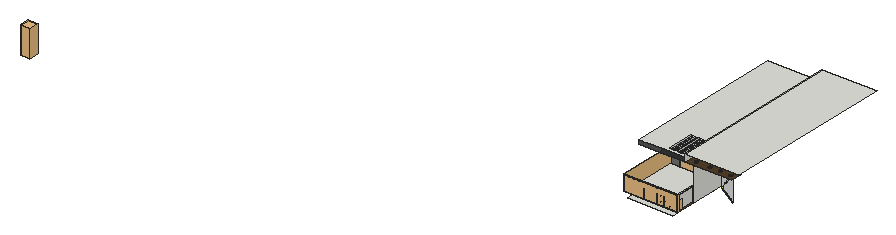
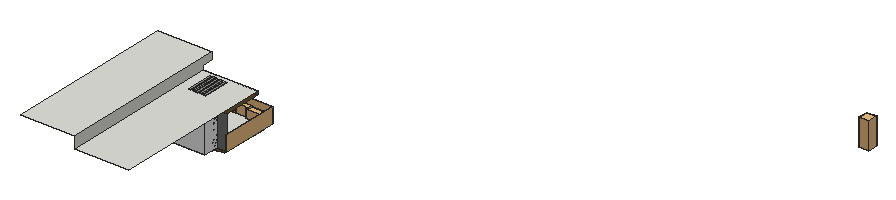
# SketchUp Ruby script. Lengths in inches.
U = 1.inch
M = Sketchup.active_model
def pt(a) = Geom::Point3d.new(a.map { |v| v * U })
def face(e, loops, mat)
  f = e.add_face(loops[0].map { |a| pt(a) })
  loops[1..].each { |l| e.add_face(l.map { |a| pt(a) }).erase! }
  f.material = f.back_material = mat if mat
  f
end
# faces: each face lists its corners as indices into pts; further lists are holes
def faces(e, pts, list, mat = nil) = list.each { |f| face(e, (f[0].is_a?(Array) ? f : [f]).map { |l| l.map { |i| pts[i] } }, mat) }
# xy, xz, yz: faces in a plane at the given z, y or x. An outline is a flat list of corners, or four numbers for a rectangle; further outlines are holes
def ring(l) = l.size == 4 ? [[l[0], l[1]], [l[2], l[1]], [l[2], l[3]], [l[0], l[3]]] : l.each_slice(2).to_a
def flat(e, list, mat, &to3) = list.each { |f| face(e, (f[0].is_a?(Array) ? f : [f]).map { |l| ring(l).map { |u, v| to3.(u, v) } }, mat) }
def xy(e, z, list, mat = nil) = flat(e, list, mat) { |x, y| [x, y, z] }
def xz(e, y, list, mat = nil) = flat(e, list, mat) { |x, z| [x, y, z] }
def yz(e, x, list, mat = nil) = flat(e, list, mat) { |y, z| [x, y, z] }
def lines(e, pts, list) = list.each { |a, b| e.add_line(pt(pts[a]), pt(pts[b])) }
# prism: a flat outline (further loops are holes) pulled along v
def prism(e, loops, v, mat = nil)
  f = face(e, loops, mat); d = Geom::Vector3d.new(v.map { |x| x * U })
  f.pushpull(f.normal.samedirection?(d) ? d.length : -d.length)
end
def box(e, o, s, mat = nil) = prism(e, [[o, [o[0] + s[0], o[1], o[2]], [o[0] + s[0], o[1] + s[1], o[2]], [o[0], o[1] + s[1], o[2]]]], [0, 0, s[2]], mat)
def at(x, y, z, deg = 0) = Geom::Transformation.translation(pt([x, y, z])) * Geom::Transformation.rotation(ORIGIN, Z_AXIS, deg.degrees)
def axes(o, x, y, z) = Geom::Transformation.new([*x, 0, *y, 0, *z, 0, *pt(o).to_a, 1])
def part(name) = M.definitions.add(name)
# library, detail: a bought-in or finely detailed component or shape, given as its bounding box
def library(name, o, s) = part(name).tap { |d| box(d.entities, o, s) }
def detail(e, o, s) = box(e.add_group.entities, o, s)
def put(e, d, t, mat = nil) = e.add_instance(d, t).tap { |i| i.material = mat if mat }
def group(e, t, mat = nil) = e.add_group.tap { |g| g.transformation = t; g.material = mat if mat }.entities
root = M.entities
M.materials.add("Concrete White 02 100cm").color = [237, 237, 237]
M.materials.add("Marble White SSS 100cm").color = [222, 222, 222]
M.materials.add("Wood Planks Pecan 33-81 150cm").color = [83, 63, 40]
M.materials.add("[Color E05]").color = [239, 239, 0]
M.materials["[Color E05]"].alpha = 0.89
M.materials.add("[Color E05]1").color = [255, 255, 0]
M.materials.add("[Color M05]").color = [114, 114, 114]
M.materials.add("[Color M06]").color = [86, 86, 86]
M.materials.add("[Color M07]").color = [58, 58, 58]
c1 = library("Planted window box",[0,0,0],[56.02,15.3,25.28])
c2 = library("Group\#2",[0,0,0],[118.08,13.29,95.4])
c3 = library("My+Glass_Railing",[-0.1,0,0],[149.63,2.52,40.9])
c4 = library("My+Glass_Railing\#1",[-0.1,0,0],[157.36,2.52,40.9])
c5 = library("30",[-486.49,477.14,411.4],[26.62,27.13,73.11])
xy(root,259.1,[[12.28,0,137.25,16.25]])
xy(root,259.1,[[[12.28,18.25,12.28,151.1875,30.69,151.1875,30.69,155.4375,118.84,155.4375,118.84,151.1875,137.25,151.1875,137.25,18.25],[123.17,35.85,124.16,35.9,125.11,36.2,125.95,36.74,126.62,37.48,127.08,38.36,127.29,39.33,127.24,40.33,126.9375,41.28,126.4,42.11,125.66,42.78,124.78,43.24,123.81,43.45,122.8125,43.4,121.87,43.1,121.03,42.5625,120.36,41.83,119.9,40.94,119.69,39.97,119.74,38.98,120.04,38.03,120.58,37.19,121.3125,36.52,122.2,36.07],[28.42,35.85,29.41,35.9,30.36,36.2,31.2,36.74,31.87,37.48,32.33,38.36,32.54,39.33,32.49,40.33,32.1875,41.28,31.65,42.11,30.91,42.78,30.03,43.24,29.06,43.45,28.0625,43.4,27.12,43.1,26.28,42.5625,25.61,41.83,25.15,40.94,24.94,39.97,24.99,38.98,25.29,38.03,25.83,37.19,26.5625,36.52,27.45,36.07],[60.17,35.85,61.16,35.9,62.11,36.2,62.95,36.74,63.62,37.48,64.08,38.36,64.29,39.33,64.24,40.33,63.9375,41.28,63.4,42.11,62.66,42.78,61.78,43.24,60.81,43.45,59.8125,43.4,58.87,43.1,58.03,42.5625,57.36,41.83,56.9,40.94,56.69,39.97,56.74,38.98,57.04,38.03,57.58,37.19,58.3125,36.52,59.2,36.07],[93.92,35.85,94.91,35.9,95.86,36.2,96.7,36.74,97.37,37.48,97.83,38.36,98.04,39.33,97.99,40.33,97.6875,41.28,97.15,42.11,96.41,42.78,95.53,43.24,94.56,43.45,93.5625,43.4,92.62,43.1,91.78,42.5625,91.11,41.83,90.65,40.94,90.44,39.97,90.49,38.98,90.79,38.03,91.33,37.19,92.0625,36.52,92.95,36.07]]],"Wood Planks Pecan 33-81 150cm")
xy(root,259.1,[[12.28,16.25,137.25,18.25]],"[Color E05]")
xy(root,271.39,[[0,0,149.53,0,149.53,1.46,146.53,1.46,146.53,54.0625,149.53,54.0625,149.53,200.375,27.125,200.375,27.125,159.875,0,159.875]])
xy(root,312.29,[[146.53,1.46,149.53,54.0625]])
xy(root,362.4,[[16.74,68.72,15.77,68.93,14.88,69.39,14.15,70.06,13.61,70.89,13.31,71.84,13.26,72.84,13.47,73.81,13.93,74.69,14.6,75.43,15.4375,75.97,16.38,76.27,17.38,76.32,18.35,76.1,19.24,75.65,19.97,74.98,20.51,74.14,20.8125,73.19,20.86,72.2,20.65,71.23,20.19,70.34,19.52,69.61,18.68,69.07,17.74,68.77],[37.18,68.72,36.21,68.93,35.32,69.39,34.59,70.06,34.05,70.89,33.75,71.84,33.7,72.84,33.91,73.81,34.37,74.69,35.04,75.43,35.875,75.97,36.82,76.27,37.82,76.32,38.79,76.1,39.67,75.65,40.41,74.98,40.95,74.14,41.25,73.19,41.3,72.2,41.08,71.23,40.63,70.34,39.96,69.61,39.12,69.07,38.17,68.77],[16.74,88.59,15.77,88.81,14.88,89.26,14.15,89.93,13.61,90.77,13.31,91.72,13.26,92.71,13.47,93.68,13.93,94.57,14.6,95.3,15.4375,95.84,16.38,96.14,17.38,96.19,18.35,95.98,19.24,95.52,19.97,94.85,20.51,94.02,20.8125,93.07,20.86,92.07,20.65,91.1,20.19,90.22,19.52,89.48,18.68,88.94,17.74,88.64],[37.18,88.59,36.21,88.81,35.32,89.26,34.59,89.93,34.05,90.77,33.75,91.72,33.7,92.71,33.91,93.68,34.37,94.57,35.04,95.3,35.875,95.84,36.82,96.14,37.82,96.19,38.79,95.98,39.67,95.52,40.41,94.85,40.95,94.02,41.25,93.07,41.3,92.07,41.08,91.1,40.63,90.22,39.96,89.48,39.12,88.94,38.17,88.64],[16.74,107.47,15.77,107.68,14.88,108.14,14.15,108.81,13.61,109.64,13.31,110.59,13.26,111.59,13.47,112.56,13.93,113.44,14.6,114.18,15.4375,114.72,16.38,115.02,17.38,115.07,18.35,114.85,19.24,114.4,19.97,113.73,20.51,112.89,20.8125,111.94,20.86,110.95,20.65,109.98,20.19,109.09,19.52,108.36,18.68,107.82,17.74,107.52],
  [37.18,107.47,36.21,107.68,35.32,108.14,34.59,108.81,34.05,109.64,33.75,110.59,33.7,111.59,33.91,112.56,34.37,113.44,35.04,114.18,35.875,114.72,36.82,115.02,37.82,115.07,38.79,114.85,39.67,114.4,40.41,113.73,40.95,112.89,41.25,111.94,41.3,110.95,41.08,109.98,40.63,109.09,39.96,108.36,39.12,107.82,38.17,107.52],[16.74,127.84,15.77,128.06,14.88,128.51,14.15,129.18,13.61,130.02,13.31,130.97,13.26,131.96,13.47,132.93,13.93,133.82,14.6,134.55,15.4375,135.09,16.38,135.39,17.38,135.44,18.35,135.23,19.24,134.77,19.97,134.1,20.51,133.27,20.8125,132.32,20.86,131.32,20.65,130.35,20.19,129.47,19.52,128.73,18.68,128.19,17.74,127.89],[37.18,127.84,36.21,128.06,35.32,128.51,34.59,129.18,34.05,130.02,33.75,130.97,33.7,131.96,33.91,132.93,34.37,133.82,35.04,134.55,35.875,135.09,36.82,135.39,37.82,135.44,38.79,135.23,39.67,134.77,40.41,134.1,40.95,133.27,41.25,132.32,41.3,131.32,41.08,130.35,40.63,129.47,39.96,128.73,39.12,128.19,38.17,127.89]])
xy(root,363.53,[[69.88,66.58,75.08,139.2],[80.28,66.58,85.48,139.2],[90.68,66.58,95.875,139.2],[101.08,66.58,106.27,139.2],[111.47,66.58,116.67,139.2],
  [121.87,66.58,126.45,139.2]])
xy(root,363.53,[[[0,54.0625,0,159.875,27.125,159.875,27.125,200.375,149.53,200.375,149.53,54.0625],[69.88,66.58,126.45,139.2],[16.74,68.72,17.74,68.77,18.68,69.07,19.52,69.61,20.19,70.34,20.65,71.23,20.86,72.2,20.8125,73.19,20.51,74.14,19.97,74.98,19.24,75.65,18.35,76.1,17.38,76.32,16.38,76.27,15.4375,75.97,14.6,75.43,13.93,74.69,13.47,73.81,13.26,72.84,13.31,71.84,13.61,70.89,14.15,70.06,14.88,69.39,15.77,68.93],[37.18,68.72,38.17,68.77,39.12,69.07,39.96,69.61,40.63,70.34,41.08,71.23,41.3,72.2,41.25,73.19,40.95,74.14,40.41,74.98,39.67,75.65,38.79,76.1,37.82,76.32,36.82,76.27,35.875,75.97,35.04,75.43,34.37,74.69,33.91,73.81,33.7,72.84,33.75,71.84,34.05,70.89,34.59,70.06,35.32,69.39,36.21,68.93],[16.74,88.59,17.74,88.64,18.68,88.94,19.52,89.48,20.19,90.22,20.65,91.1,20.86,92.07,20.8125,93.07,20.51,94.02,19.97,94.85,19.24,95.52,18.35,95.98,17.38,96.19,16.38,96.14,15.4375,95.84,14.6,95.3,13.93,94.57,13.47,93.68,13.26,92.71,13.31,91.72,13.61,90.77,14.15,89.93,14.88,89.26,15.77,88.81],[37.18,88.59,38.17,88.64,39.12,88.94,39.96,89.48,40.63,90.22,41.08,91.1,41.3,92.07,41.25,93.07,40.95,94.02,40.41,94.85,39.67,95.52,38.79,95.98,37.82,96.19,36.82,96.14,35.875,95.84,35.04,95.3,34.37,94.57,33.91,93.68,33.7,92.71,33.75,91.72,34.05,90.77,34.59,89.93,35.32,89.26,36.21,88.81],[16.74,107.47,17.74,107.52,18.68,107.82,19.52,108.36,20.19,109.09,20.65,109.98,20.86,110.95,20.8125,111.94,20.51,112.89,19.97,113.73,19.24,114.4,18.35,114.85,17.38,115.07,16.38,115.02,15.4375,114.72,14.6,114.18,13.93,113.44,13.47,112.56,13.26,111.59,13.31,110.59,13.61,109.64,14.15,108.81,14.88,108.14,15.77,107.68],[37.18,107.47,38.17,107.52,39.12,107.82,39.96,108.36,40.63,109.09,41.08,109.98,41.3,110.95,41.25,111.94,40.95,112.89,40.41,113.73,39.67,114.4,38.79,114.85,37.82,115.07,36.82,115.02,35.875,114.72,35.04,114.18,34.37,113.44,33.91,112.56,33.7,111.59,33.75,110.59,34.05,109.64,34.59,108.81,35.32,108.14,36.21,107.68],[16.74,127.84,17.74,127.89,18.68,128.19,19.52,128.73,20.19,129.47,20.65,130.35,20.86,131.32,20.8125,132.32,20.51,133.27,19.97,134.1,19.24,134.77,18.35,135.23,17.38,135.44,16.38,135.39,15.4375,135.09,14.6,134.55,13.93,133.82,13.47,132.93,13.26,131.96,13.31,130.97,13.61,130.02,14.15,129.18,14.88,128.51,15.77,128.06],[37.18,127.84,38.17,127.89,39.12,128.19,39.96,128.73,40.63,129.47,41.08,130.35,41.3,131.32,41.25,132.32,40.95,133.27,40.41,134.1,39.67,134.77,38.79,135.23,37.82,135.44,36.82,135.39,35.875,135.09,35.04,134.55,34.37,133.82,33.91,132.93,33.7,131.96,33.75,130.97,34.05,130.02,34.59,129.18,35.32,128.51,36.21,128.06]]],"Wood Planks Pecan 33-81 150cm")
xy(root,374.3125,[[[0,54.0625,149.53,497],[75.08,66.58,80.28,139.2],[85.48,66.58,90.68,139.2],[95.875,66.58,101.08,139.2],[106.27,66.58,111.47,139.2],[116.67,66.58,121.87,139.2]]])
xy(root,383.79,[[168.59,36.78,167.62,36.99,166.73,37.45,166,38.12,165.46,38.95,165.16,39.9,165.11,40.9,165.32,41.87,165.78,42.75,166.45,43.49,167.29,44.03,168.23,44.33,169.23,44.375,170.2,44.16,171.08,43.71,171.82,43.04,172.36,42.2,172.66,41.25,172.71,40.26,172.5,39.29,172.04,38.4,171.37,37.66,170.53,37.13,169.58,36.82],[205.47,36.78,204.49,36.99,203.61,37.45,202.87,38.12,202.33,38.95,202.03,39.9,201.98,40.9,202.2,41.87,202.65,42.75,203.32,43.49,204.16,44.03,205.11,44.33,206.1,44.375,207.08,44.16,207.96,43.71,208.7,43.04,209.23,42.2,209.54,41.25,209.58,40.26,209.37,39.29,208.91,38.4,208.24,37.66,207.41,37.13,206.46,36.82],[234.09,36.78,233.12,36.99,232.23,37.45,231.5,38.12,230.96,38.95,230.66,39.9,230.61,40.9,230.82,41.87,231.28,42.75,231.95,43.49,232.79,44.03,233.73,44.33,234.73,44.375,235.7,44.16,236.58,43.71,237.32,43.04,237.86,42.2,238.16,41.25,238.21,40.26,238,39.29,237.54,38.4,236.87,37.66,236.03,37.13,235.08,36.82],[263.34,36.78,262.37,36.99,261.48,37.45,260.75,38.12,260.21,38.95,259.91,39.9,259.86,40.9,260.07,41.87,260.53,42.75,261.2,43.49,262.04,44.03,262.98,44.33,263.98,44.375,264.95,44.16,265.83,43.71,266.57,43.04,267.11,42.2,267.41,41.25,267.46,40.26,267.25,39.29,266.79,38.4,266.12,37.66,265.28,37.13,264.33,36.82]])
xy(root,384.73,[[[149.53,25.125,279.23,54.0625],[263.34,36.78,264.33,36.82,265.28,37.13,266.12,37.66,266.79,38.4,267.25,39.29,267.46,40.26,267.41,41.25,267.11,42.2,266.57,43.04,265.83,43.71,264.95,44.16,263.98,44.375,262.98,44.33,262.04,44.03,261.2,43.49,260.53,42.75,260.07,41.87,259.86,40.9,259.91,39.9,260.21,38.95,260.75,38.12,261.48,37.45,262.37,36.99],[168.59,36.78,169.58,36.82,170.53,37.13,171.37,37.66,172.04,38.4,172.5,39.29,172.71,40.26,172.66,41.25,172.36,42.2,171.82,43.04,171.08,43.71,170.2,44.16,169.23,44.375,168.23,44.33,167.29,44.03,166.45,43.49,165.78,42.75,165.32,41.87,165.11,40.9,165.16,39.9,165.46,38.95,166,38.12,166.73,37.45,167.62,36.99],[205.47,36.78,206.46,36.82,207.41,37.13,208.24,37.66,208.91,38.4,209.37,39.29,209.58,40.26,209.54,41.25,209.23,42.2,208.7,43.04,207.96,43.71,207.08,44.16,206.1,44.375,205.11,44.33,204.16,44.03,203.32,43.49,202.65,42.75,202.2,41.87,201.98,40.9,202.03,39.9,202.33,38.95,202.87,38.12,203.61,37.45,204.49,36.99],[234.09,36.78,235.08,36.82,236.03,37.13,236.87,37.66,237.54,38.4,238,39.29,238.21,40.26,238.16,41.25,237.86,42.2,237.32,43.04,236.58,43.71,235.7,44.16,234.73,44.375,233.73,44.33,232.79,44.03,231.95,43.49,231.28,42.75,230.82,41.87,230.61,40.9,230.66,39.9,230.96,38.95,231.5,38.12,232.23,37.45,233.12,36.99]]],"Wood Planks Pecan 33-81 150cm")
xy(root,404.5625,[[149.53,25.125,299.0625,497]])
xz(root,1.46,[[146.53,271.39,149.53,312.29]])
xz(root,54.0625,[[146.53,271.39,149.53,312.29]])
xz(root,54.0625,[[257.84,311.67,257.84,380.95,229.74,335.16],[227.16,334.74,257.84,384.73,227.16,384.73]],"Marble White SSS 100cm")
xz(root,54.0625,[[257.84,309.1,257.84,311.67,229.74,335.16,257.84,380.95,257.84,384.73,227.16,334.74]],"[Color E05]1")
xz(root,54.0625,[[0,363.53,59.94,374.3125]],"[Color M06]")
xz(root,54.0625,[[59.94,363.53,149.53,374.3125]],"[Color M07]")
xz(root,66.58,[[75.08,363.53,80.28,374.3125],[85.48,363.53,90.68,374.3125],[95.875,363.53,101.08,374.3125],[106.27,363.53,111.47,374.3125],[116.67,363.53,121.87,374.3125]])
xz(root,139.2,[[75.08,363.53,80.28,374.3125],[85.48,363.53,90.68,374.3125],[95.875,363.53,101.08,374.3125],[106.27,363.53,111.47,374.3125],[116.67,363.53,121.87,374.3125]])
xz(root,159.875,[[0,271.39,27.125,363.53]],"[Color M05]")
xz(root,200.375,[[27.125,271.39,149.53,363.53]],"Concrete White 02 100cm")
yz(root,27.125,[[159.875,271.39,200.375,363.53]],"Concrete White 02 100cm")
yz(root,75.08,[[66.58,363.53,139.2,374.3125]])
yz(root,80.28,[[66.58,363.53,139.2,374.3125]])
yz(root,85.48,[[66.58,363.53,139.2,374.3125]])
yz(root,90.68,[[66.58,363.53,139.2,374.3125]])
yz(root,95.875,[[66.58,363.53,139.2,374.3125]])
yz(root,101.08,[[66.58,363.53,139.2,374.3125]])
yz(root,106.27,[[66.58,363.53,139.2,374.3125]])
yz(root,111.47,[[66.58,363.53,139.2,374.3125]])
yz(root,116.67,[[66.58,363.53,139.2,374.3125]])
yz(root,121.87,[[66.58,363.53,139.2,374.3125]])
yz(root,146.53,[[1.46,271.39,54.0625,312.29]])
yz(root,149.53,[[54.0625,271.39,200.375,363.53],[54.0625,374.3125,54.0625,384.73,25.125,384.73,25.125,404.5625,497,404.5625,497,374.3125]])
p = [[16.74,68.72,363.53],[15.77,68.93,363.53],[15.77,68.93,362.4],[16.74,68.72,362.4],[17.74,68.77,363.53],[17.74,68.77,362.4],
  [37.18,68.72,363.53],[36.21,68.93,363.53],[36.21,68.93,362.4],[37.18,68.72,362.4],[38.17,68.77,363.53],[38.17,68.77,362.4],
  [18.68,69.07,363.53],[18.68,69.07,362.4],[39.12,69.07,363.53],[39.12,69.07,362.4],[14.88,69.39,363.53],[14.88,69.39,362.4],
  [35.32,69.39,363.53],[35.32,69.39,362.4],[19.52,69.61,363.53],[19.52,69.61,362.4],[39.96,69.61,363.53],[39.96,69.61,362.4],
  [14.15,70.06,363.53],[14.15,70.06,362.4],[34.59,70.06,363.53],[34.59,70.06,362.4],[20.19,70.34,363.53],[20.19,70.34,362.4],
  [40.63,70.34,363.53],[40.63,70.34,362.4],[13.61,70.89,363.53],[13.61,70.89,362.4],[34.05,70.89,363.53],[34.05,70.89,362.4],
  [20.65,71.23,363.53],[20.65,71.23,362.4],[41.08,71.23,363.53],[41.08,71.23,362.4],[13.31,71.84,363.53],[13.31,71.84,362.4],
  [33.75,71.84,363.53],[33.75,71.84,362.4],[20.86,72.2,363.53],[20.86,72.2,362.4],[41.3,72.2,363.53],[41.3,72.2,362.4],
  [13.26,72.84,363.53],[13.26,72.84,362.4],[33.7,72.84,363.53],[33.7,72.84,362.4],[20.8125,73.19,363.53],[20.8125,73.19,362.4],
  [41.25,73.19,363.53],[41.25,73.19,362.4],[13.47,73.81,363.53],[13.47,73.81,362.4],[33.91,73.81,363.53],[33.91,73.81,362.4],
  [20.51,74.14,363.53],[20.51,74.14,362.4],[40.95,74.14,363.53],[40.95,74.14,362.4],[13.93,74.69,363.53],[13.93,74.69,362.4],
  [34.37,74.69,363.53],[34.37,74.69,362.4],[19.97,74.98,363.53],[19.97,74.98,362.4],[40.41,74.98,363.53],[40.41,74.98,362.4],
  [14.6,75.43,363.53],[14.6,75.43,362.4],[35.04,75.43,363.53],[35.04,75.43,362.4],[19.24,75.65,363.53],[19.24,75.65,362.4],
  [39.67,75.65,363.53],[39.67,75.65,362.4],[15.4375,75.97,363.53],[15.4375,75.97,362.4],[35.875,75.97,363.53],[35.875,75.97,362.4],
  [18.35,76.1,363.53],[18.35,76.1,362.4],[38.79,76.1,363.53],[38.79,76.1,362.4],[16.38,76.27,363.53],[16.38,76.27,362.4],
  [36.82,76.27,363.53],[36.82,76.27,362.4],[17.38,76.32,363.53],[17.38,76.32,362.4],[37.82,76.32,363.53],[37.82,76.32,362.4],
  [16.74,88.59,363.53],[15.77,88.81,363.53],[15.77,88.81,362.4],[16.74,88.59,362.4],[17.74,88.64,363.53],[17.74,88.64,362.4],
  [18.68,88.94,363.53],[18.68,88.94,362.4],[37.18,88.59,363.53],[36.21,88.81,363.53],[36.21,88.81,362.4],[37.18,88.59,362.4],
  [38.17,88.64,363.53],[38.17,88.64,362.4],[39.12,88.94,363.53],[39.12,88.94,362.4],[14.88,89.26,363.53],[14.88,89.26,362.4],
  [35.32,89.26,363.53],[35.32,89.26,362.4],[19.52,89.48,363.53],[19.52,89.48,362.4],[39.96,89.48,363.53],[39.96,89.48,362.4],
  [14.15,89.93,363.53],[14.15,89.93,362.4],[34.59,89.93,363.53],[34.59,89.93,362.4],[20.19,90.22,363.53],[20.19,90.22,362.4],
  [40.63,90.22,363.53],[40.63,90.22,362.4],[13.61,90.77,363.53],[13.61,90.77,362.4],[34.05,90.77,363.53],[34.05,90.77,362.4],
  [20.65,91.1,363.53],[20.65,91.1,362.4],[41.08,91.1,363.53],[41.08,91.1,362.4],[13.31,91.72,363.53],[13.31,91.72,362.4],
  [33.75,91.72,363.53],[33.75,91.72,362.4],[20.86,92.07,363.53],[20.86,92.07,362.4],[41.3,92.07,363.53],[41.3,92.07,362.4],
  [13.26,92.71,363.53],[13.26,92.71,362.4],[33.7,92.71,363.53],[33.7,92.71,362.4],[20.8125,93.07,363.53],[20.8125,93.07,362.4],
  [41.25,93.07,363.53],[41.25,93.07,362.4],[13.47,93.68,363.53],[13.47,93.68,362.4],[33.91,93.68,363.53],[33.91,93.68,362.4],
  [20.51,94.02,363.53],[20.51,94.02,362.4],[40.95,94.02,363.53],[40.95,94.02,362.4],[13.93,94.57,363.53],[13.93,94.57,362.4],
  [34.37,94.57,363.53],[34.37,94.57,362.4],[19.97,94.85,363.53],[19.97,94.85,362.4],[40.41,94.85,363.53],[40.41,94.85,362.4],
  [14.6,95.3,363.53],[14.6,95.3,362.4],[35.04,95.3,363.53],[35.04,95.3,362.4],[19.24,95.52,363.53],[19.24,95.52,362.4],
  [39.67,95.52,363.53],[39.67,95.52,362.4],[15.4375,95.84,363.53],[15.4375,95.84,362.4],[35.875,95.84,363.53],[35.875,95.84,362.4],
  [18.35,95.98,363.53],[18.35,95.98,362.4],[38.79,95.98,363.53],[38.79,95.98,362.4],[16.38,96.14,363.53],[16.38,96.14,362.4],
  [36.82,96.14,363.53],[36.82,96.14,362.4],[17.38,96.19,363.53],[17.38,96.19,362.4],[37.82,96.19,363.53],[37.82,96.19,362.4],
  [16.74,107.47,363.53],[15.77,107.68,363.53],[15.77,107.68,362.4],[16.74,107.47,362.4],[17.74,107.52,363.53],[17.74,107.52,362.4],
  [18.68,107.82,363.53],[18.68,107.82,362.4],[37.18,107.47,363.53],[36.21,107.68,363.53],[36.21,107.68,362.4],[37.18,107.47,362.4],
  [38.17,107.52,363.53],[38.17,107.52,362.4],[39.12,107.82,363.53],[39.12,107.82,362.4],[14.88,108.14,363.53],[14.88,108.14,362.4],
  [35.32,108.14,363.53],[35.32,108.14,362.4],[19.52,108.36,363.53],[19.52,108.36,362.4],[39.96,108.36,363.53],[39.96,108.36,362.4],
  [14.15,108.81,363.53],[14.15,108.81,362.4],[34.59,108.81,363.53],[34.59,108.81,362.4],[20.19,109.09,363.53],[20.19,109.09,362.4],
  [40.63,109.09,363.53],[40.63,109.09,362.4],[13.61,109.64,363.53],[13.61,109.64,362.4],[34.05,109.64,363.53],[34.05,109.64,362.4],
  [20.65,109.98,363.53],[20.65,109.98,362.4],[41.08,109.98,363.53],[41.08,109.98,362.4],[13.31,110.59,363.53],[13.31,110.59,362.4],
  [33.75,110.59,363.53],[33.75,110.59,362.4],[20.86,110.95,363.53],[20.86,110.95,362.4],[41.3,110.95,363.53],[41.3,110.95,362.4],
  [13.26,111.59,363.53],[13.26,111.59,362.4],[33.7,111.59,363.53],[33.7,111.59,362.4],[20.8125,111.94,363.53],[20.8125,111.94,362.4],
  [41.25,111.94,363.53],[41.25,111.94,362.4],[13.47,112.56,363.53],[13.47,112.56,362.4],[33.91,112.56,363.53],[33.91,112.56,362.4],
  [20.51,112.89,363.53],[20.51,112.89,362.4],[40.95,112.89,363.53],[40.95,112.89,362.4],[13.93,113.44,363.53],[13.93,113.44,362.4],
  [34.37,113.44,363.53],[34.37,113.44,362.4],[19.97,113.73,363.53],[19.97,113.73,362.4],[40.41,113.73,363.53],[40.41,113.73,362.4],
  [14.6,114.18,363.53],[14.6,114.18,362.4],[35.04,114.18,363.53],[35.04,114.18,362.4],[19.24,114.4,363.53],[19.24,114.4,362.4],
  [39.67,114.4,363.53],[39.67,114.4,362.4],[15.4375,114.72,363.53],[15.4375,114.72,362.4],[35.875,114.72,363.53],[35.875,114.72,362.4],
  [18.35,114.85,363.53],[18.35,114.85,362.4],[38.79,114.85,363.53],[38.79,114.85,362.4],[16.38,115.02,363.53],[16.38,115.02,362.4],
  [36.82,115.02,363.53],[36.82,115.02,362.4],[17.38,115.07,363.53],[17.38,115.07,362.4],[37.82,115.07,363.53],[37.82,115.07,362.4],
  [16.74,127.84,363.53],[15.77,128.06,363.53],[15.77,128.06,362.4],[16.74,127.84,362.4],[17.74,127.89,363.53],[17.74,127.89,362.4],
  [37.18,127.84,363.53],[36.21,128.06,363.53],[36.21,128.06,362.4],[37.18,127.84,362.4],[38.17,127.89,363.53],[38.17,127.89,362.4],
  [18.68,128.19,363.53],[18.68,128.19,362.4],[39.12,128.19,363.53],[39.12,128.19,362.4],[14.88,128.51,363.53],[14.88,128.51,362.4],
  [35.32,128.51,363.53],[35.32,128.51,362.4],[19.52,128.73,363.53],[19.52,128.73,362.4],[39.96,128.73,363.53],[39.96,128.73,362.4],
  [14.15,129.18,363.53],[14.15,129.18,362.4],[34.59,129.18,363.53],[34.59,129.18,362.4],[20.19,129.47,363.53],[20.19,129.47,362.4],
  [40.63,129.47,363.53],[40.63,129.47,362.4],[13.61,130.02,363.53],[13.61,130.02,362.4],[34.05,130.02,363.53],[34.05,130.02,362.4],
  [20.65,130.35,363.53],[20.65,130.35,362.4],[41.08,130.35,363.53],[41.08,130.35,362.4],[13.31,130.97,363.53],[13.31,130.97,362.4],
  [33.75,130.97,363.53],[33.75,130.97,362.4],[20.86,131.32,363.53],[20.86,131.32,362.4],[41.3,131.32,363.53],[41.3,131.32,362.4],
  [13.26,131.96,363.53],[13.26,131.96,362.4],[33.7,131.96,363.53],[33.7,131.96,362.4],[20.8125,132.32,363.53],[20.8125,132.32,362.4],
  [41.25,132.32,363.53],[41.25,132.32,362.4],[13.47,132.93,363.53],[13.47,132.93,362.4],[33.91,132.93,363.53],[33.91,132.93,362.4],
  [20.51,133.27,363.53],[20.51,133.27,362.4],[40.95,133.27,363.53],[40.95,133.27,362.4],[13.93,133.82,363.53],[13.93,133.82,362.4],
  [34.37,133.82,363.53],[34.37,133.82,362.4],[19.97,134.1,363.53],[19.97,134.1,362.4],[40.41,134.1,363.53],[40.41,134.1,362.4],
  [14.6,134.55,363.53],[14.6,134.55,362.4],[35.04,134.55,363.53],[35.04,134.55,362.4],[19.24,134.77,363.53],[19.24,134.77,362.4],
  [39.67,134.77,363.53],[39.67,134.77,362.4],[15.4375,135.09,363.53],[15.4375,135.09,362.4],[35.875,135.09,363.53],[35.875,135.09,362.4],
  [18.35,135.23,363.53],[18.35,135.23,362.4],[38.79,135.23,363.53],[38.79,135.23,362.4],[16.38,135.39,363.53],[16.38,135.39,362.4],
  [36.82,135.39,363.53],[36.82,135.39,362.4],[17.38,135.44,363.53],[17.38,135.44,362.4],[37.82,135.44,363.53],[37.82,135.44,362.4],
  [168.59,36.78,384.73],[167.62,36.99,384.73],[167.62,36.99,383.79],[168.59,36.78,383.79],[169.58,36.82,384.73],[169.58,36.82,383.79],
  [170.53,37.13,384.73],[170.53,37.13,383.79],[205.47,36.78,384.73],[204.49,36.99,384.73],[204.49,36.99,383.79],[205.47,36.78,383.79],
  [206.46,36.82,384.73],[206.46,36.82,383.79],[207.41,37.13,384.73],[207.41,37.13,383.79],[234.09,36.78,384.73],[233.12,36.99,384.73],
  [233.12,36.99,383.79],[234.09,36.78,383.79],[235.08,36.82,384.73],[235.08,36.82,383.79],[236.03,37.13,384.73],[236.03,37.13,383.79],
  [263.34,36.78,384.73],[262.37,36.99,384.73],[262.37,36.99,383.79],[263.34,36.78,383.79],[264.33,36.82,384.73],[264.33,36.82,383.79],
  [265.28,37.13,384.73],[265.28,37.13,383.79],[166.73,37.45,384.73],[166.73,37.45,383.79],[203.61,37.45,384.73],[203.61,37.45,383.79],
  [232.23,37.45,384.73],[232.23,37.45,383.79],[261.48,37.45,384.73],[261.48,37.45,383.79],[171.37,37.66,384.73],[171.37,37.66,383.79],
  [208.24,37.66,384.73],[208.24,37.66,383.79],[236.87,37.66,384.73],[236.87,37.66,383.79],[266.12,37.66,384.73],[266.12,37.66,383.79],
  [166,38.12,384.73],[166,38.12,383.79],[202.87,38.12,384.73],[202.87,38.12,383.79],[231.5,38.12,384.73],[231.5,38.12,383.79],
  [260.75,38.12,384.73],[260.75,38.12,383.79],[172.04,38.4,384.73],[172.04,38.4,383.79],[208.91,38.4,384.73],[208.91,38.4,383.79],
  [237.54,38.4,384.73],[237.54,38.4,383.79],[266.79,38.4,384.73],[266.79,38.4,383.79],[165.46,38.95,384.73],[165.46,38.95,383.79],
  [202.33,38.95,384.73],[202.33,38.95,383.79],[230.96,38.95,384.73],[230.96,38.95,383.79],[260.21,38.95,384.73],[260.21,38.95,383.79],
  [172.5,39.29,384.73],[172.5,39.29,383.79],[209.37,39.29,384.73],[209.37,39.29,383.79],[238,39.29,384.73],[238,39.29,383.79],
  [267.25,39.29,384.73],[267.25,39.29,383.79],[165.16,39.9,384.73],[165.16,39.9,383.79],[202.03,39.9,384.73],[202.03,39.9,383.79],
  [230.66,39.9,384.73],[230.66,39.9,383.79],[259.91,39.9,384.73],[259.91,39.9,383.79],[172.71,40.26,384.73],[172.71,40.26,383.79],
  [209.58,40.26,384.73],[209.58,40.26,383.79],[238.21,40.26,384.73],[238.21,40.26,383.79],[267.46,40.26,384.73],[267.46,40.26,383.79],
  [165.11,40.9,384.73],[165.11,40.9,383.79],[201.98,40.9,384.73],[201.98,40.9,383.79],[230.61,40.9,384.73],[230.61,40.9,383.79],
  [259.86,40.9,384.73],[259.86,40.9,383.79],[172.66,41.25,384.73],[172.66,41.25,383.79],[209.54,41.25,384.73],[209.54,41.25,383.79],
  [238.16,41.25,384.73],[238.16,41.25,383.79],[267.41,41.25,384.73],[267.41,41.25,383.79],[165.32,41.87,384.73],[165.32,41.87,383.79],
  [202.2,41.87,384.73],[202.2,41.87,383.79],[230.82,41.87,384.73],[230.82,41.87,383.79],[260.07,41.87,384.73],[260.07,41.87,383.79],
  [172.36,42.2,384.73],[172.36,42.2,383.79],[209.23,42.2,384.73],[209.23,42.2,383.79],[237.86,42.2,384.73],[237.86,42.2,383.79],
  [267.11,42.2,384.73],[267.11,42.2,383.79],[165.78,42.75,384.73],[165.78,42.75,383.79],[202.65,42.75,384.73],[202.65,42.75,383.79],
  [231.28,42.75,384.73],[231.28,42.75,383.79],[260.53,42.75,384.73],[260.53,42.75,383.79],[171.82,43.04,384.73],[171.82,43.04,383.79],
  [208.7,43.04,384.73],[208.7,43.04,383.79],[237.32,43.04,384.73],[237.32,43.04,383.79],[266.57,43.04,384.73],[266.57,43.04,383.79],
  [166.45,43.49,384.73],[166.45,43.49,383.79],[203.32,43.49,384.73],[203.32,43.49,383.79],[231.95,43.49,384.73],[231.95,43.49,383.79],
  [261.2,43.49,384.73],[261.2,43.49,383.79],[171.08,43.71,384.73],[171.08,43.71,383.79],[207.96,43.71,384.73],[207.96,43.71,383.79],
  [236.58,43.71,384.73],[236.58,43.71,383.79],[265.83,43.71,384.73],[265.83,43.71,383.79],[167.29,44.03,384.73],[167.29,44.03,383.79],
  [204.16,44.03,384.73],[204.16,44.03,383.79],[232.79,44.03,384.73],[232.79,44.03,383.79],[262.04,44.03,384.73],[262.04,44.03,383.79],
  [170.2,44.16,384.73],[170.2,44.16,383.79],[207.08,44.16,384.73],[207.08,44.16,383.79],[235.7,44.16,384.73],[235.7,44.16,383.79],
  [264.95,44.16,384.73],[264.95,44.16,383.79],[168.23,44.33,384.73],[168.23,44.33,383.79],[205.11,44.33,384.73],[205.11,44.33,383.79],
  [233.73,44.33,384.73],[233.73,44.33,383.79],[262.98,44.33,384.73],[262.98,44.33,383.79],[169.23,44.375,384.73],[169.23,44.375,383.79],
  [206.1,44.375,384.73],[206.1,44.375,383.79],[234.73,44.375,384.73],[234.73,44.375,383.79],[263.98,44.375,384.73],[263.98,44.375,383.79],
  [257.84,54.0625,380.95],[259.38,54.0625,383.45]]
faces(root,p,[[0,1,2,3],[4,0,3,5],[6,7,8,9],[10,6,9,11],[12,4,5,13],[14,10,11,15],[1,16,17,2],[7,18,19,8],
  [20,12,13,21],[22,14,15,23],[16,24,25,17],[18,26,27,19],[28,20,21,29],[30,22,23,31],[24,32,33,25],[26,34,35,27],
  [36,28,29,37],[38,30,31,39],[32,40,41,33],[34,42,43,35],[44,36,37,45],[46,38,39,47],[40,48,49,41],[42,50,51,43],
  [52,44,45,53],[54,46,47,55],[48,56,57,49],[50,58,59,51],[60,52,53,61],[62,54,55,63],[56,64,65,57],[58,66,67,59],
  [68,60,61,69],[70,62,63,71],[64,72,73,65],[66,74,75,67],[76,68,69,77],[78,70,71,79],[72,80,81,73],[74,82,83,75],
  [84,76,77,85],[86,78,79,87],[80,88,89,81],[82,90,91,83],[92,84,85,93],[94,86,87,95],[88,92,93,89],[90,94,95,91],
  [96,97,98,99],[100,96,99,101],[102,100,101,103],[104,105,106,107],[108,104,107,109],[110,108,109,111],[97,112,113,98],[105,114,115,106],
  [116,102,103,117],[118,110,111,119],[112,120,121,113],[114,122,123,115],[124,116,117,125],[126,118,119,127],[120,128,129,121],[122,130,131,123],
  [132,124,125,133],[134,126,127,135],[128,136,137,129],[130,138,139,131],[140,132,133,141],[142,134,135,143],[136,144,145,137],[138,146,147,139],
  [148,140,141,149],[150,142,143,151],[144,152,153,145],[146,154,155,147],[156,148,149,157],[158,150,151,159],[152,160,161,153],[154,162,163,155],
  [164,156,157,165],[166,158,159,167],[160,168,169,161],[162,170,171,163],[172,164,165,173],[174,166,167,175],[168,176,177,169],[170,178,179,171],
  [180,172,173,181],[182,174,175,183],[176,184,185,177],[178,186,187,179],[188,180,181,189],[190,182,183,191],[184,188,189,185],[186,190,191,187],
  [192,193,194,195],[196,192,195,197],[198,196,197,199],[200,201,202,203],[204,200,203,205],[206,204,205,207],[193,208,209,194],[201,210,211,202],
  [212,198,199,213],[214,206,207,215],[208,216,217,209],[210,218,219,211],[220,212,213,221],[222,214,215,223],[216,224,225,217],[218,226,227,219],
  [228,220,221,229],[230,222,223,231],[224,232,233,225],[226,234,235,227],[236,228,229,237],[238,230,231,239],[232,240,241,233],[234,242,243,235],
  [244,236,237,245],[246,238,239,247],[240,248,249,241],[242,250,251,243],[252,244,245,253],[254,246,247,255],[248,256,257,249],[250,258,259,251],
  [260,252,253,261],[262,254,255,263],[256,264,265,257],[258,266,267,259],[268,260,261,269],[270,262,263,271],[264,272,273,265],[266,274,275,267],
  [276,268,269,277],[278,270,271,279],[272,280,281,273],[274,282,283,275],[284,276,277,285],[286,278,279,287],[280,284,285,281],[282,286,287,283],
  [288,289,290,291],[292,288,291,293],[294,295,296,297],[298,294,297,299],[300,292,293,301],[302,298,299,303],[289,304,305,290],[295,306,307,296],
  [308,300,301,309],[310,302,303,311],[304,312,313,305],[306,314,315,307],[316,308,309,317],[318,310,311,319],[312,320,321,313],[314,322,323,315],
  [324,316,317,325],[326,318,319,327],[320,328,329,321],[322,330,331,323],[332,324,325,333],[334,326,327,335],[328,336,337,329],[330,338,339,331],
  [340,332,333,341],[342,334,335,343],[336,344,345,337],[338,346,347,339],[348,340,341,349],[350,342,343,351],[344,352,353,345],[346,354,355,347],
  [356,348,349,357],[358,350,351,359],[352,360,361,353],[354,362,363,355],[364,356,357,365],[366,358,359,367],[360,368,369,361],[362,370,371,363],
  [372,364,365,373],[374,366,367,375],[368,376,377,369],[370,378,379,371],[380,372,373,381],[382,374,375,383],[376,380,381,377],[378,382,383,379],
  [384,385,386,387],[388,384,387,389],[390,388,389,391],[392,393,394,395],[396,392,395,397],[398,396,397,399],[400,401,402,403],[404,400,403,405],
  [406,404,405,407],[408,409,410,411],[412,408,411,413],[414,412,413,415],[385,416,417,386],[393,418,419,394],[401,420,421,402],[409,422,423,410],
  [424,390,391,425],[426,398,399,427],[428,406,407,429],[430,414,415,431],[416,432,433,417],[418,434,435,419],[420,436,437,421],[422,438,439,423],
  [440,424,425,441],[442,426,427,443],[444,428,429,445],[446,430,431,447],[432,448,449,433],[434,450,451,435],[436,452,453,437],[438,454,455,439],
  [456,440,441,457],[458,442,443,459],[460,444,445,461],[462,446,447,463],[448,464,465,449],[450,466,467,451],[452,468,469,453],[454,470,471,455],
  [472,456,457,473],[474,458,459,475],[476,460,461,477],[478,462,463,479],[464,480,481,465],[466,482,483,467],[468,484,485,469],[470,486,487,471],
  [488,472,473,489],[490,474,475,491],[492,476,477,493],[494,478,479,495],[480,496,497,481],[482,498,499,483],[484,500,501,485],[486,502,503,487],
  [504,488,489,505],[506,490,491,507],[508,492,493,509],[510,494,495,511],[496,512,513,497],[498,514,515,499],[500,516,517,501],[502,518,519,503],
  [520,504,505,521],[522,506,507,523],[524,508,509,525],[526,510,511,527],[512,528,529,513],[514,530,531,515],[516,532,533,517],[518,534,535,519],
  [536,520,521,537],[538,522,523,539],[540,524,525,541],[542,526,527,543],[528,544,545,529],[530,546,547,531],[532,548,549,533],[534,550,551,535],
  [552,536,537,553],[554,538,539,555],[556,540,541,557],[558,542,543,559],[544,560,561,545],[546,562,563,547],[548,564,565,549],[550,566,567,551],
  [568,552,553,569],[570,554,555,571],[572,556,557,573],[574,558,559,575],[560,568,569,561],[562,570,571,563],[564,572,573,565],[566,574,575,567]])
lines(root,p,[[576,577]])
put(root,c1,at(4.61,4.23,268.9))
put(root,c2,axes([27.125,159.875,270.04],[1,0,0],[0,1,0],[0,0,0.98]))
put(root,c3,at(0,0,271.39))
put(root,c1,at(55.8125,0,271.39))
put(root,c1,at(92.0625,0,271.39))
put(root,c4,at(-0.1,159.77,271.4,-90))
put(root,c5,at(-744.61,-1014.73,0))
